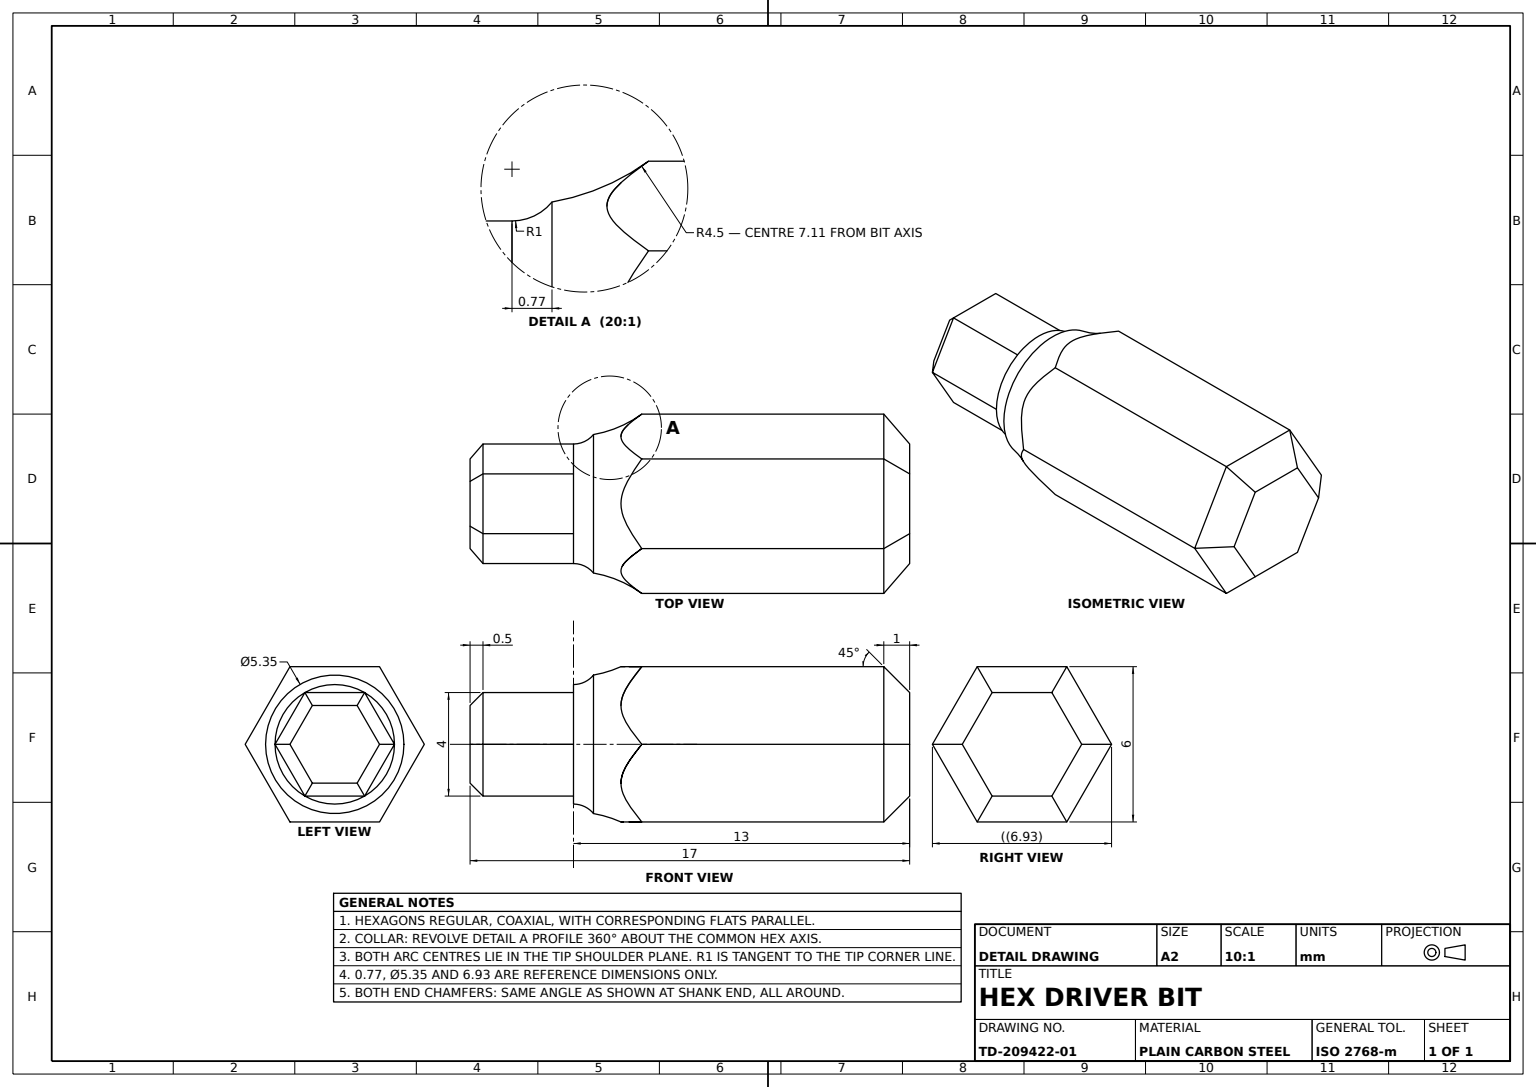
ISO-10303-21;
HEADER;
FILE_DESCRIPTION((''),'2;1');
FILE_NAME('','',(''),(''),'','','');
FILE_SCHEMA(('AUTOMOTIVE_DESIGN'));
ENDSEC;
DATA;
#1=APPLICATION_CONTEXT('');
#2=PRODUCT_CONTEXT('',#1,'mechanical');
#3=PRODUCT('','','',(#2));
#4=PRODUCT_DEFINITION_FORMATION('','',#3);
#5=PRODUCT_DEFINITION_CONTEXT('',#1,'design');
#6=PRODUCT_DEFINITION('','',#4,#5);
#7=PRODUCT_DEFINITION_SHAPE('','',#6);
#8=(LENGTH_UNIT()NAMED_UNIT(*)SI_UNIT(.MILLI.,.METRE.));
#9=(NAMED_UNIT(*)PLANE_ANGLE_UNIT()SI_UNIT($,.RADIAN.));
#10=(NAMED_UNIT(*)SI_UNIT($,.STERADIAN.)SOLID_ANGLE_UNIT());
#11=UNCERTAINTY_MEASURE_WITH_UNIT(LENGTH_MEASURE(1.E-05),#8,'distance_accuracy_value','');
#12=(GEOMETRIC_REPRESENTATION_CONTEXT(3)GLOBAL_UNCERTAINTY_ASSIGNED_CONTEXT((#11))GLOBAL_UNIT_ASSIGNED_CONTEXT((#8,#9,#10))REPRESENTATION_CONTEXT('',''));
#13=CARTESIAN_POINT('',(-2.67534,0.,12.226717));
#14=VERTEX_POINT('',#13);
#15=CARTESIAN_POINT('',(-2.309401,0.,13.));
#16=VERTEX_POINT('',#15);
#17=CARTESIAN_POINT('',(-3.309401,0.,13.));
#18=DIRECTION('',(0.,-1.,0.));
#19=DIRECTION('',(0.,0.,-1.));
#20=AXIS2_PLACEMENT_3D('',#17,#18,#19);
#21=CIRCLE('',#20,1.);
#22=EDGE_CURVE('',#14,#16,#21,.T.);
#23=ORIENTED_EDGE('',*,*,#22,.F.);
#24=CARTESIAN_POINT('',(2.67534,0.,12.226717));
#25=VERTEX_POINT('',#24);
#26=CARTESIAN_POINT('',(0.,0.,12.226717));
#27=DIRECTION('',(-1.,0.,0.));
#28=AXIS2_PLACEMENT_3D('',#26,#19,#27);
#29=CIRCLE('',#28,2.67534);
#30=EDGE_CURVE('',#25,#14,#29,.T.);
#31=ORIENTED_EDGE('',*,*,#30,.F.);
#32=CARTESIAN_POINT('',(2.309401,0.,13.));
#33=VERTEX_POINT('',#32);
#34=CARTESIAN_POINT('',(3.309401,0.,13.));
#35=DIRECTION('',(0.,1.,0.));
#36=AXIS2_PLACEMENT_3D('',#34,#35,#27);
#37=CIRCLE('',#36,1.);
#38=EDGE_CURVE('',#25,#33,#37,.T.);
#39=ORIENTED_EDGE('',*,*,#38,.T.);
#40=CARTESIAN_POINT('',(1.154701,-2.,13.));
#41=VERTEX_POINT('',#40);
#42=CARTESIAN_POINT('',(0.,0.,13.));
#43=AXIS2_PLACEMENT_3D('',#42,#19,#27);
#44=CIRCLE('',#43,2.309401);
#45=EDGE_CURVE('',#33,#41,#44,.T.);
#46=ORIENTED_EDGE('',*,*,#45,.T.);
#47=CARTESIAN_POINT('',(-1.154701,-2.,13.));
#48=VERTEX_POINT('',#47);
#49=EDGE_CURVE('',#41,#48,#44,.T.);
#50=ORIENTED_EDGE('',*,*,#49,.T.);
#51=EDGE_CURVE('',#48,#16,#44,.T.);
#52=ORIENTED_EDGE('',*,*,#51,.T.);
#53=EDGE_LOOP('',(#23,#31,#39,#46,#50,#52));
#54=FACE_OUTER_BOUND('',#53,.T.);
#55=TOROIDAL_SURFACE('',#43,3.309401,1.);
#56=ADVANCED_FACE('',(#54),#55,.F.);
#57=ORIENTED_EDGE('',*,*,#51,.F.);
#58=CARTESIAN_POINT('',(-1.732051,-1.,13.));
#59=DIRECTION('',(0.5,-0.866025404,0.));
#60=VECTOR('',#59,1000.);
#61=LINE('',#58,#60);
#62=EDGE_CURVE('',#16,#48,#61,.T.);
#63=ORIENTED_EDGE('',*,*,#62,.F.);
#64=EDGE_LOOP('',(#57,#63));
#65=FACE_OUTER_BOUND('',#64,.T.);
#66=DIRECTION('',(0.,0.,1.));
#67=DIRECTION('',(1.,0.,0.));
#68=AXIS2_PLACEMENT_3D('',#42,#66,#67);
#69=PLANE('',#68);
#70=ADVANCED_FACE('',(#65),#69,.T.);
#71=CARTESIAN_POINT('',(-0.866025,-1.5,17.));
#72=VERTEX_POINT('',#71);
#73=CARTESIAN_POINT('',(-1.154701,-2.,16.5));
#74=VERTEX_POINT('',#73);
#75=CARTESIAN_POINT('',(-0.742307,-1.285714,17.214286));
#76=DIRECTION('',(-0.377964473,-0.654653671,-0.654653671));
#77=VECTOR('',#76,1000.);
#78=LINE('',#75,#77);
#79=EDGE_CURVE('',#72,#74,#78,.T.);
#80=ORIENTED_EDGE('',*,*,#79,.F.);
#81=CARTESIAN_POINT('',(-1.732051,0.,17.));
#82=VERTEX_POINT('',#81);
#83=CARTESIAN_POINT('',(-1.299038,-0.75,17.));
#84=LINE('',#83,#60);
#85=EDGE_CURVE('',#82,#72,#84,.T.);
#86=ORIENTED_EDGE('',*,*,#85,.F.);
#87=CARTESIAN_POINT('',(-2.309401,0.,16.5));
#88=VERTEX_POINT('',#87);
#89=CARTESIAN_POINT('',(-1.484615,0.,17.214286));
#90=DIRECTION('',(-0.755928946,0.,-0.654653671));
#91=VECTOR('',#90,1000.);
#92=LINE('',#89,#91);
#93=EDGE_CURVE('',#82,#88,#92,.T.);
#94=ORIENTED_EDGE('',*,*,#93,.T.);
#95=DIRECTION('',(-0.5,0.866025404,0.));
#96=VECTOR('',#95,1000.);
#97=LINE('',#87,#96);
#98=EDGE_CURVE('',#74,#88,#97,.T.);
#99=ORIENTED_EDGE('',*,*,#98,.F.);
#100=EDGE_LOOP('',(#80,#86,#94,#99));
#101=FACE_OUTER_BOUND('',#100,.T.);
#102=DIRECTION('',(0.612372436,0.353553391,-0.707106781));
#103=AXIS2_PLACEMENT_3D('',#83,#102,#59);
#104=PLANE('',#103);
#105=ADVANCED_FACE('',(#101),#104,.F.);
#106=CARTESIAN_POINT('',(1.732051,3.,10.360098));
#107=VERTEX_POINT('',#106);
#108=CARTESIAN_POINT('',(-1.732051,3.,10.360098));
#109=VERTEX_POINT('',#108);
#110=CARTESIAN_POINT('',(1.46548,3.,10.544095));
#111=CARTESIAN_POINT('',(1.199534,3.,10.729064));
#112=CARTESIAN_POINT('',(0.772596,3.,10.962951));
#113=CARTESIAN_POINT('',(0.626195,3.,11.032542));
#114=CARTESIAN_POINT('',(0.319103,3.,11.134062));
#115=CARTESIAN_POINT('',(0.157579,3.,11.164407));
#116=CARTESIAN_POINT('',(-0.165078,3.,11.163504));
#117=CARTESIAN_POINT('',(-0.327037,3.,11.132159));
#118=CARTESIAN_POINT('',(-0.634019,3.,11.029198));
#119=CARTESIAN_POINT('',(-0.781209,3.,10.958587));
#120=CARTESIAN_POINT('',(-1.203607,3.,10.726096));
#121=CARTESIAN_POINT('',(-1.467558,3.,10.54266));
#122=B_SPLINE_CURVE_WITH_KNOTS('',3,(#106,#110,#111,#112,#113,#114,#115,#116,#117,#118,#119,#120,#121,#108),.UNSPECIFIED.,.F.,.F.,(4,2,2,2,2,2,4),(0.004347057,0.005310347,0.005791992,0.006273637,0.006755282,0.007236927,0.008200217),.UNSPECIFIED.);
#123=EDGE_CURVE('',#107,#109,#122,.T.);
#124=ORIENTED_EDGE('',*,*,#123,.F.);
#125=CARTESIAN_POINT('',(1.732051,3.,1.));
#126=VERTEX_POINT('',#125);
#127=CARTESIAN_POINT('',(1.732051,3.,13.));
#128=VECTOR('',#19,1000.);
#129=LINE('',#127,#128);
#130=EDGE_CURVE('',#107,#126,#129,.T.);
#131=ORIENTED_EDGE('',*,*,#130,.T.);
#132=CARTESIAN_POINT('',(-1.732051,3.,1.));
#133=VERTEX_POINT('',#132);
#134=VECTOR('',#27,1000.);
#135=LINE('',#125,#134);
#136=EDGE_CURVE('',#126,#133,#135,.T.);
#137=ORIENTED_EDGE('',*,*,#136,.T.);
#138=CARTESIAN_POINT('',(-1.732051,3.,13.));
#139=LINE('',#138,#128);
#140=EDGE_CURVE('',#109,#133,#139,.T.);
#141=ORIENTED_EDGE('',*,*,#140,.F.);
#142=EDGE_LOOP('',(#124,#131,#137,#141));
#143=FACE_OUTER_BOUND('',#142,.T.);
#144=AXIS2_PLACEMENT_3D('',#127,#18,#19);
#145=PLANE('',#144);
#146=ADVANCED_FACE('',(#143),#145,.F.);
#147=CARTESIAN_POINT('',(0.866025,1.5,17.));
#148=VERTEX_POINT('',#147);
#149=CARTESIAN_POINT('',(-0.866025,1.5,17.));
#150=VERTEX_POINT('',#149);
#151=CARTESIAN_POINT('',(0.,1.5,17.));
#152=LINE('',#151,#134);
#153=EDGE_CURVE('',#148,#150,#152,.T.);
#154=ORIENTED_EDGE('',*,*,#153,.F.);
#155=CARTESIAN_POINT('',(1.154701,2.,16.5));
#156=VERTEX_POINT('',#155);
#157=CARTESIAN_POINT('',(0.742307,1.285714,17.214286));
#158=DIRECTION('',(-0.377964473,-0.654653671,0.654653671));
#159=VECTOR('',#158,1000.);
#160=LINE('',#157,#159);
#161=EDGE_CURVE('',#156,#148,#160,.T.);
#162=ORIENTED_EDGE('',*,*,#161,.F.);
#163=CARTESIAN_POINT('',(-1.154701,2.,16.5));
#164=VERTEX_POINT('',#163);
#165=VECTOR('',#67,1000.);
#166=LINE('',#155,#165);
#167=EDGE_CURVE('',#164,#156,#166,.T.);
#168=ORIENTED_EDGE('',*,*,#167,.F.);
#169=CARTESIAN_POINT('',(-0.742307,1.285714,17.214286));
#170=DIRECTION('',(-0.377964473,0.654653671,-0.654653671));
#171=VECTOR('',#170,1000.);
#172=LINE('',#169,#171);
#173=EDGE_CURVE('',#150,#164,#172,.T.);
#174=ORIENTED_EDGE('',*,*,#173,.F.);
#175=EDGE_LOOP('',(#154,#162,#168,#174));
#176=FACE_OUTER_BOUND('',#175,.T.);
#177=DIRECTION('',(0.,-0.707106781,-0.707106781));
#178=AXIS2_PLACEMENT_3D('',#151,#177,#27);
#179=PLANE('',#178);
#180=ADVANCED_FACE('',(#176),#179,.F.);
#181=CARTESIAN_POINT('',(2.309401,0.,16.5));
#182=VERTEX_POINT('',#181);
#183=LINE('',#181,#60);
#184=EDGE_CURVE('',#156,#182,#183,.T.);
#185=ORIENTED_EDGE('',*,*,#184,.F.);
#186=ORIENTED_EDGE('',*,*,#161,.T.);
#187=CARTESIAN_POINT('',(1.732051,0.,17.));
#188=VERTEX_POINT('',#187);
#189=CARTESIAN_POINT('',(1.299038,0.75,17.));
#190=LINE('',#189,#96);
#191=EDGE_CURVE('',#188,#148,#190,.T.);
#192=ORIENTED_EDGE('',*,*,#191,.F.);
#193=CARTESIAN_POINT('',(1.484615,0.,17.214286));
#194=DIRECTION('',(-0.755928946,0.,0.654653671));
#195=VECTOR('',#194,1000.);
#196=LINE('',#193,#195);
#197=EDGE_CURVE('',#182,#188,#196,.T.);
#198=ORIENTED_EDGE('',*,*,#197,.F.);
#199=EDGE_LOOP('',(#185,#186,#192,#198));
#200=FACE_OUTER_BOUND('',#199,.T.);
#201=DIRECTION('',(-0.612372436,-0.353553391,-0.707106781));
#202=AXIS2_PLACEMENT_3D('',#189,#201,#95);
#203=PLANE('',#202);
#204=ADVANCED_FACE('',(#200),#203,.F.);
#205=CARTESIAN_POINT('',(-1.154701,2.,13.));
#206=VERTEX_POINT('',#205);
#207=CARTESIAN_POINT('',(-1.732051,1.,13.));
#208=DIRECTION('',(-0.5,-0.866025404,0.));
#209=VECTOR('',#208,1000.);
#210=LINE('',#207,#209);
#211=EDGE_CURVE('',#206,#16,#210,.T.);
#212=ORIENTED_EDGE('',*,*,#211,.F.);
#213=EDGE_CURVE('',#16,#206,#44,.T.);
#214=ORIENTED_EDGE('',*,*,#213,.F.);
#215=EDGE_LOOP('',(#212,#214));
#216=FACE_OUTER_BOUND('',#215,.T.);
#217=ADVANCED_FACE('',(#216),#69,.T.);
#218=CARTESIAN_POINT('',(-1.154701,2.,0.));
#219=VERTEX_POINT('',#218);
#220=CARTESIAN_POINT('',(1.154701,2.,0.));
#221=VERTEX_POINT('',#220);
#222=CARTESIAN_POINT('',(0.,2.,0.));
#223=LINE('',#222,#165);
#224=EDGE_CURVE('',#219,#221,#223,.T.);
#225=ORIENTED_EDGE('',*,*,#224,.T.);
#226=CARTESIAN_POINT('',(2.309401,0.,0.));
#227=VERTEX_POINT('',#226);
#228=CARTESIAN_POINT('',(1.732051,1.,0.));
#229=LINE('',#228,#60);
#230=EDGE_CURVE('',#221,#227,#229,.T.);
#231=ORIENTED_EDGE('',*,*,#230,.T.);
#232=CARTESIAN_POINT('',(1.154701,-2.,0.));
#233=VERTEX_POINT('',#232);
#234=CARTESIAN_POINT('',(1.732051,-1.,0.));
#235=LINE('',#234,#209);
#236=EDGE_CURVE('',#227,#233,#235,.T.);
#237=ORIENTED_EDGE('',*,*,#236,.T.);
#238=CARTESIAN_POINT('',(-1.154701,-2.,0.));
#239=VERTEX_POINT('',#238);
#240=CARTESIAN_POINT('',(0.,-2.,0.));
#241=LINE('',#240,#134);
#242=EDGE_CURVE('',#233,#239,#241,.T.);
#243=ORIENTED_EDGE('',*,*,#242,.T.);
#244=CARTESIAN_POINT('',(-2.309401,0.,0.));
#245=VERTEX_POINT('',#244);
#246=CARTESIAN_POINT('',(-1.732051,-1.,0.));
#247=LINE('',#246,#96);
#248=EDGE_CURVE('',#239,#245,#247,.T.);
#249=ORIENTED_EDGE('',*,*,#248,.T.);
#250=CARTESIAN_POINT('',(-1.732051,1.,0.));
#251=DIRECTION('',(0.5,0.866025404,0.));
#252=VECTOR('',#251,1000.);
#253=LINE('',#250,#252);
#254=EDGE_CURVE('',#245,#219,#253,.T.);
#255=ORIENTED_EDGE('',*,*,#254,.T.);
#256=EDGE_LOOP('',(#225,#231,#237,#243,#249,#255));
#257=FACE_OUTER_BOUND('',#256,.T.);
#258=CARTESIAN_POINT('',(0.,0.,0.));
#259=AXIS2_PLACEMENT_3D('',#258,#66,#67);
#260=PLANE('',#259);
#261=ADVANCED_FACE('',(#257),#260,.F.);
#262=ORIENTED_EDGE('',*,*,#173,.T.);
#263=LINE('',#163,#252);
#264=EDGE_CURVE('',#88,#164,#263,.T.);
#265=ORIENTED_EDGE('',*,*,#264,.F.);
#266=ORIENTED_EDGE('',*,*,#93,.F.);
#267=CARTESIAN_POINT('',(-1.299038,0.75,17.));
#268=LINE('',#267,#209);
#269=EDGE_CURVE('',#150,#82,#268,.T.);
#270=ORIENTED_EDGE('',*,*,#269,.F.);
#271=EDGE_LOOP('',(#262,#265,#266,#270));
#272=FACE_OUTER_BOUND('',#271,.T.);
#273=DIRECTION('',(0.612372436,-0.353553391,-0.707106781));
#274=AXIS2_PLACEMENT_3D('',#267,#273,#208);
#275=PLANE('',#274);
#276=ADVANCED_FACE('',(#272),#275,.F.);
#277=CARTESIAN_POINT('',(1.154701,-2.,16.5));
#278=VERTEX_POINT('',#277);
#279=LINE('',#277,#209);
#280=EDGE_CURVE('',#182,#278,#279,.T.);
#281=ORIENTED_EDGE('',*,*,#280,.F.);
#282=ORIENTED_EDGE('',*,*,#197,.T.);
#283=CARTESIAN_POINT('',(0.866025,-1.5,17.));
#284=VERTEX_POINT('',#283);
#285=CARTESIAN_POINT('',(1.299038,-0.75,17.));
#286=LINE('',#285,#252);
#287=EDGE_CURVE('',#284,#188,#286,.T.);
#288=ORIENTED_EDGE('',*,*,#287,.F.);
#289=CARTESIAN_POINT('',(0.742307,-1.285714,17.214286));
#290=DIRECTION('',(-0.377964473,0.654653671,0.654653671));
#291=VECTOR('',#290,1000.);
#292=LINE('',#289,#291);
#293=EDGE_CURVE('',#278,#284,#292,.T.);
#294=ORIENTED_EDGE('',*,*,#293,.F.);
#295=EDGE_LOOP('',(#281,#282,#288,#294));
#296=FACE_OUTER_BOUND('',#295,.T.);
#297=DIRECTION('',(-0.612372436,0.353553391,-0.707106781));
#298=AXIS2_PLACEMENT_3D('',#285,#297,#251);
#299=PLANE('',#298);
#300=ADVANCED_FACE('',(#296),#299,.F.);
#301=CARTESIAN_POINT('',(-1.732051,-3.,10.360098));
#302=VERTEX_POINT('',#301);
#303=CARTESIAN_POINT('',(1.732051,-3.,10.360098));
#304=VERTEX_POINT('',#303);
#305=CARTESIAN_POINT('',(-1.46548,-3.,10.544095));
#306=CARTESIAN_POINT('',(-1.199534,-3.,10.729064));
#307=CARTESIAN_POINT('',(-0.772596,-3.,10.962951));
#308=CARTESIAN_POINT('',(-0.626195,-3.,11.032542));
#309=CARTESIAN_POINT('',(-0.319103,-3.,11.134062));
#310=CARTESIAN_POINT('',(-0.157579,-3.,11.164407));
#311=CARTESIAN_POINT('',(0.165078,-3.,11.163504));
#312=CARTESIAN_POINT('',(0.327037,-3.,11.132159));
#313=CARTESIAN_POINT('',(0.634019,-3.,11.029198));
#314=CARTESIAN_POINT('',(0.781209,-3.,10.958587));
#315=CARTESIAN_POINT('',(1.203607,-3.,10.726096));
#316=CARTESIAN_POINT('',(1.467558,-3.,10.54266));
#317=B_SPLINE_CURVE_WITH_KNOTS('',3,(#301,#305,#306,#307,#308,#309,#310,#311,#312,#313,#314,#315,#316,#303),.UNSPECIFIED.,.F.,.F.,(4,2,2,2,2,2,4),(0.004347057,0.005310347,0.005791992,0.006273637,0.006755282,0.007236927,0.008200217),.UNSPECIFIED.);
#318=EDGE_CURVE('',#302,#304,#317,.T.);
#319=ORIENTED_EDGE('',*,*,#318,.F.);
#320=CARTESIAN_POINT('',(-1.732051,-3.,1.));
#321=VERTEX_POINT('',#320);
#322=CARTESIAN_POINT('',(-1.732051,-3.,13.));
#323=LINE('',#322,#128);
#324=EDGE_CURVE('',#302,#321,#323,.T.);
#325=ORIENTED_EDGE('',*,*,#324,.T.);
#326=CARTESIAN_POINT('',(1.732051,-3.,1.));
#327=VERTEX_POINT('',#326);
#328=LINE('',#320,#165);
#329=EDGE_CURVE('',#321,#327,#328,.T.);
#330=ORIENTED_EDGE('',*,*,#329,.T.);
#331=CARTESIAN_POINT('',(1.732051,-3.,13.));
#332=LINE('',#331,#128);
#333=EDGE_CURVE('',#304,#327,#332,.T.);
#334=ORIENTED_EDGE('',*,*,#333,.F.);
#335=EDGE_LOOP('',(#319,#325,#330,#334));
#336=FACE_OUTER_BOUND('',#335,.T.);
#337=AXIS2_PLACEMENT_3D('',#322,#35,#66);
#338=PLANE('',#337);
#339=ADVANCED_FACE('',(#336),#338,.F.);
#340=CARTESIAN_POINT('',(1.154701,2.,13.));
#341=VERTEX_POINT('',#340);
#342=EDGE_CURVE('',#341,#33,#44,.T.);
#343=ORIENTED_EDGE('',*,*,#342,.F.);
#344=CARTESIAN_POINT('',(1.732051,1.,13.));
#345=LINE('',#344,#96);
#346=EDGE_CURVE('',#33,#341,#345,.T.);
#347=ORIENTED_EDGE('',*,*,#346,.F.);
#348=EDGE_LOOP('',(#343,#347));
#349=FACE_OUTER_BOUND('',#348,.T.);
#350=ADVANCED_FACE('',(#349),#69,.T.);
#351=CARTESIAN_POINT('',(-3.464102,0.,10.360098));
#352=VERTEX_POINT('',#351);
#353=CARTESIAN_POINT('',(-1.865194,2.76939,10.543898));
#354=CARTESIAN_POINT('',(-1.99824,2.538946,10.728897));
#355=CARTESIAN_POINT('',(-2.211152,2.170172,10.96231));
#356=CARTESIAN_POINT('',(-2.283891,2.044184,11.031576));
#357=CARTESIAN_POINT('',(-2.436992,1.779005,11.133292));
#358=CARTESIAN_POINT('',(-2.517802,1.639038,11.164022));
#359=CARTESIAN_POINT('',(-2.678865,1.360069,11.163899));
#360=CARTESIAN_POINT('',(-2.759942,1.219639,11.132945));
#361=CARTESIAN_POINT('',(-2.913333,0.953959,11.030688));
#362=CARTESIAN_POINT('',(-2.987069,0.826245,10.960215));
#363=CARTESIAN_POINT('',(-3.198866,0.459402,10.7275));
#364=CARTESIAN_POINT('',(-3.331351,0.229931,10.543357));
#365=B_SPLINE_CURVE_WITH_KNOTS('',3,(#108,#353,#354,#355,#356,#357,#358,#359,#360,#361,#362,#363,#364,#351),.UNSPECIFIED.,.F.,.F.,(4,2,2,2,2,2,4),(0.00000028,0.000970506,0.001455618,0.001940731,0.002425844,0.002910956,0.003881181),.UNSPECIFIED.);
#366=EDGE_CURVE('',#109,#352,#365,.T.);
#367=ORIENTED_EDGE('',*,*,#366,.T.);
#368=CARTESIAN_POINT('',(-7.108401,0.,13.));
#369=AXIS2_PLACEMENT_3D('',#368,#18,#19);
#370=CIRCLE('',#369,4.5);
#371=EDGE_CURVE('',#352,#14,#370,.T.);
#372=ORIENTED_EDGE('',*,*,#371,.T.);
#373=EDGE_CURVE('',#14,#25,#29,.T.);
#374=ORIENTED_EDGE('',*,*,#373,.T.);
#375=CARTESIAN_POINT('',(3.464102,0.,10.360098));
#376=VERTEX_POINT('',#375);
#377=CARTESIAN_POINT('',(7.108401,0.,13.));
#378=AXIS2_PLACEMENT_3D('',#377,#35,#27);
#379=CIRCLE('',#378,4.5);
#380=EDGE_CURVE('',#376,#25,#379,.T.);
#381=ORIENTED_EDGE('',*,*,#380,.F.);
#382=CARTESIAN_POINT('',(3.330959,0.23061,10.543898));
#383=CARTESIAN_POINT('',(3.197912,0.461054,10.728897));
#384=CARTESIAN_POINT('',(2.985,0.829828,10.96231));
#385=CARTESIAN_POINT('',(2.912261,0.955816,11.031576));
#386=CARTESIAN_POINT('',(2.75916,1.220995,11.133292));
#387=CARTESIAN_POINT('',(2.67835,1.360962,11.164022));
#388=CARTESIAN_POINT('',(2.517287,1.639931,11.163899));
#389=CARTESIAN_POINT('',(2.43621,1.780361,11.132945));
#390=CARTESIAN_POINT('',(2.282819,2.046041,11.030688));
#391=CARTESIAN_POINT('',(2.209083,2.173755,10.960215));
#392=CARTESIAN_POINT('',(1.997287,2.540598,10.7275));
#393=CARTESIAN_POINT('',(1.864802,2.770069,10.543357));
#394=B_SPLINE_CURVE_WITH_KNOTS('',3,(#375,#382,#383,#384,#385,#386,#387,#388,#389,#390,#391,#392,#393,#106),.UNSPECIFIED.,.F.,.F.,(4,2,2,2,2,2,4),(0.00000028,0.000970506,0.001455618,0.001940731,0.002425844,0.002910956,0.003881181),.UNSPECIFIED.);
#395=EDGE_CURVE('',#376,#107,#394,.T.);
#396=ORIENTED_EDGE('',*,*,#395,.T.);
#397=ORIENTED_EDGE('',*,*,#123,.T.);
#398=EDGE_LOOP('',(#367,#372,#374,#381,#396,#397));
#399=FACE_OUTER_BOUND('',#398,.T.);
#400=TOROIDAL_SURFACE('',#43,7.108401,4.5);
#401=ADVANCED_FACE('',(#399),#400,.F.);
#402=CARTESIAN_POINT('',(-1.154701,-2.,9.));
#403=VECTOR('',#66,1000.);
#404=LINE('',#402,#403);
#405=EDGE_CURVE('',#48,#74,#404,.T.);
#406=ORIENTED_EDGE('',*,*,#405,.T.);
#407=ORIENTED_EDGE('',*,*,#98,.T.);
#408=CARTESIAN_POINT('',(-2.309401,0.,9.));
#409=LINE('',#408,#403);
#410=EDGE_CURVE('',#16,#88,#409,.T.);
#411=ORIENTED_EDGE('',*,*,#410,.F.);
#412=ORIENTED_EDGE('',*,*,#62,.T.);
#413=EDGE_LOOP('',(#406,#407,#411,#412));
#414=FACE_OUTER_BOUND('',#413,.T.);
#415=DIRECTION('',(-0.866025404,-0.5,0.));
#416=AXIS2_PLACEMENT_3D('',#408,#415,#59);
#417=PLANE('',#416);
#418=ADVANCED_FACE('',(#414),#417,.T.);
#419=ORIENTED_EDGE('',*,*,#136,.F.);
#420=DIRECTION('',(0.377964473,0.654653671,0.654653671));
#421=VECTOR('',#420,1000.);
#422=LINE('',#125,#421);
#423=EDGE_CURVE('',#221,#126,#422,.T.);
#424=ORIENTED_EDGE('',*,*,#423,.F.);
#425=ORIENTED_EDGE('',*,*,#224,.F.);
#426=LINE('',#132,#291);
#427=EDGE_CURVE('',#219,#133,#426,.T.);
#428=ORIENTED_EDGE('',*,*,#427,.T.);
#429=EDGE_LOOP('',(#419,#424,#425,#428));
#430=FACE_OUTER_BOUND('',#429,.T.);
#431=DIRECTION('',(0.,-0.707106781,0.707106781));
#432=AXIS2_PLACEMENT_3D('',#125,#431,#27);
#433=PLANE('',#432);
#434=ADVANCED_FACE('',(#430),#433,.F.);
#435=CARTESIAN_POINT('',(3.464102,0.,1.));
#436=VERTEX_POINT('',#435);
#437=LINE('',#326,#252);
#438=EDGE_CURVE('',#327,#436,#437,.T.);
#439=ORIENTED_EDGE('',*,*,#438,.T.);
#440=CARTESIAN_POINT('',(3.464102,0.,13.));
#441=LINE('',#440,#128);
#442=EDGE_CURVE('',#376,#436,#441,.T.);
#443=ORIENTED_EDGE('',*,*,#442,.F.);
#444=CARTESIAN_POINT('',(1.865194,-2.76939,10.543898));
#445=CARTESIAN_POINT('',(1.99824,-2.538946,10.728897));
#446=CARTESIAN_POINT('',(2.211152,-2.170172,10.96231));
#447=CARTESIAN_POINT('',(2.283891,-2.044184,11.031576));
#448=CARTESIAN_POINT('',(2.436992,-1.779005,11.133292));
#449=CARTESIAN_POINT('',(2.517802,-1.639038,11.164022));
#450=CARTESIAN_POINT('',(2.678865,-1.360069,11.163899));
#451=CARTESIAN_POINT('',(2.759942,-1.219639,11.132945));
#452=CARTESIAN_POINT('',(2.913333,-0.953959,11.030688));
#453=CARTESIAN_POINT('',(2.987069,-0.826245,10.960215));
#454=CARTESIAN_POINT('',(3.198866,-0.459402,10.7275));
#455=CARTESIAN_POINT('',(3.331351,-0.229931,10.543357));
#456=B_SPLINE_CURVE_WITH_KNOTS('',3,(#303,#444,#445,#446,#447,#448,#449,#450,#451,#452,#453,#454,#455,#375),.UNSPECIFIED.,.F.,.F.,(4,2,2,2,2,2,4),(0.00000028,0.000970506,0.001455618,0.001940731,0.002425844,0.002910956,0.003881181),.UNSPECIFIED.);
#457=EDGE_CURVE('',#304,#376,#456,.T.);
#458=ORIENTED_EDGE('',*,*,#457,.F.);
#459=ORIENTED_EDGE('',*,*,#333,.T.);
#460=EDGE_LOOP('',(#439,#443,#458,#459));
#461=FACE_OUTER_BOUND('',#460,.T.);
#462=DIRECTION('',(-0.866025404,0.5,0.));
#463=AXIS2_PLACEMENT_3D('',#331,#462,#208);
#464=PLANE('',#463);
#465=ADVANCED_FACE('',(#461),#464,.F.);
#466=ORIENTED_EDGE('',*,*,#329,.F.);
#467=DIRECTION('',(0.377964473,0.654653671,-0.654653671));
#468=VECTOR('',#467,1000.);
#469=LINE('',#320,#468);
#470=EDGE_CURVE('',#321,#239,#469,.T.);
#471=ORIENTED_EDGE('',*,*,#470,.T.);
#472=ORIENTED_EDGE('',*,*,#242,.F.);
#473=LINE('',#326,#171);
#474=EDGE_CURVE('',#327,#233,#473,.T.);
#475=ORIENTED_EDGE('',*,*,#474,.F.);
#476=EDGE_LOOP('',(#466,#471,#472,#475));
#477=FACE_OUTER_BOUND('',#476,.T.);
#478=DIRECTION('',(0.,0.707106781,0.707106781));
#479=AXIS2_PLACEMENT_3D('',#320,#478,#67);
#480=PLANE('',#479);
#481=ADVANCED_FACE('',(#477),#480,.F.);
#482=ORIENTED_EDGE('',*,*,#427,.F.);
#483=ORIENTED_EDGE('',*,*,#254,.F.);
#484=CARTESIAN_POINT('',(-3.464102,0.,1.));
#485=VERTEX_POINT('',#484);
#486=LINE('',#484,#195);
#487=EDGE_CURVE('',#245,#485,#486,.T.);
#488=ORIENTED_EDGE('',*,*,#487,.T.);
#489=LINE('',#132,#209);
#490=EDGE_CURVE('',#133,#485,#489,.T.);
#491=ORIENTED_EDGE('',*,*,#490,.F.);
#492=EDGE_LOOP('',(#482,#483,#488,#491));
#493=FACE_OUTER_BOUND('',#492,.T.);
#494=DIRECTION('',(0.612372436,-0.353553391,0.707106781));
#495=AXIS2_PLACEMENT_3D('',#132,#494,#208);
#496=PLANE('',#495);
#497=ADVANCED_FACE('',(#493),#496,.F.);
#498=ORIENTED_EDGE('',*,*,#474,.T.);
#499=ORIENTED_EDGE('',*,*,#236,.F.);
#500=CARTESIAN_POINT('',(2.474358,0.,0.142857));
#501=LINE('',#500,#91);
#502=EDGE_CURVE('',#436,#227,#501,.T.);
#503=ORIENTED_EDGE('',*,*,#502,.F.);
#504=ORIENTED_EDGE('',*,*,#438,.F.);
#505=EDGE_LOOP('',(#498,#499,#503,#504));
#506=FACE_OUTER_BOUND('',#505,.T.);
#507=DIRECTION('',(-0.612372436,0.353553391,0.707106781));
#508=AXIS2_PLACEMENT_3D('',#326,#507,#251);
#509=PLANE('',#508);
#510=ADVANCED_FACE('',(#506),#509,.F.);
#511=ORIENTED_EDGE('',*,*,#167,.T.);
#512=CARTESIAN_POINT('',(1.154701,2.,9.));
#513=LINE('',#512,#403);
#514=EDGE_CURVE('',#341,#156,#513,.T.);
#515=ORIENTED_EDGE('',*,*,#514,.F.);
#516=CARTESIAN_POINT('',(0.,2.,13.));
#517=LINE('',#516,#134);
#518=EDGE_CURVE('',#341,#206,#517,.T.);
#519=ORIENTED_EDGE('',*,*,#518,.T.);
#520=CARTESIAN_POINT('',(-1.154701,2.,9.));
#521=LINE('',#520,#403);
#522=EDGE_CURVE('',#206,#164,#521,.T.);
#523=ORIENTED_EDGE('',*,*,#522,.T.);
#524=EDGE_LOOP('',(#511,#515,#519,#523));
#525=FACE_OUTER_BOUND('',#524,.T.);
#526=AXIS2_PLACEMENT_3D('',#512,#35,#66);
#527=PLANE('',#526);
#528=ADVANCED_FACE('',(#525),#527,.T.);
#529=ORIENTED_EDGE('',*,*,#85,.T.);
#530=CARTESIAN_POINT('',(0.,-1.5,17.));
#531=LINE('',#530,#165);
#532=EDGE_CURVE('',#72,#284,#531,.T.);
#533=ORIENTED_EDGE('',*,*,#532,.T.);
#534=ORIENTED_EDGE('',*,*,#287,.T.);
#535=ORIENTED_EDGE('',*,*,#191,.T.);
#536=ORIENTED_EDGE('',*,*,#153,.T.);
#537=ORIENTED_EDGE('',*,*,#269,.T.);
#538=EDGE_LOOP('',(#529,#533,#534,#535,#536,#537));
#539=FACE_OUTER_BOUND('',#538,.T.);
#540=CARTESIAN_POINT('',(0.,0.,17.));
#541=AXIS2_PLACEMENT_3D('',#540,#66,#67);
#542=PLANE('',#541);
#543=ADVANCED_FACE('',(#539),#542,.T.);
#544=CARTESIAN_POINT('',(-3.464102,0.,13.));
#545=LINE('',#544,#128);
#546=EDGE_CURVE('',#352,#485,#545,.T.);
#547=ORIENTED_EDGE('',*,*,#546,.F.);
#548=ORIENTED_EDGE('',*,*,#366,.F.);
#549=ORIENTED_EDGE('',*,*,#140,.T.);
#550=ORIENTED_EDGE('',*,*,#490,.T.);
#551=EDGE_LOOP('',(#547,#548,#549,#550));
#552=FACE_OUTER_BOUND('',#551,.T.);
#553=DIRECTION('',(0.866025404,-0.5,0.));
#554=AXIS2_PLACEMENT_3D('',#138,#553,#251);
#555=PLANE('',#554);
#556=ADVANCED_FACE('',(#552),#555,.F.);
#557=ORIENTED_EDGE('',*,*,#342,.T.);
#558=ORIENTED_EDGE('',*,*,#38,.F.);
#559=ORIENTED_EDGE('',*,*,#373,.F.);
#560=ORIENTED_EDGE('',*,*,#22,.T.);
#561=ORIENTED_EDGE('',*,*,#213,.T.);
#562=EDGE_CURVE('',#206,#341,#44,.T.);
#563=ORIENTED_EDGE('',*,*,#562,.T.);
#564=EDGE_LOOP('',(#557,#558,#559,#560,#561,#563));
#565=FACE_OUTER_BOUND('',#564,.T.);
#566=ADVANCED_FACE('',(#565),#55,.F.);
#567=ORIENTED_EDGE('',*,*,#45,.F.);
#568=CARTESIAN_POINT('',(1.732051,-1.,13.));
#569=LINE('',#568,#252);
#570=EDGE_CURVE('',#41,#33,#569,.T.);
#571=ORIENTED_EDGE('',*,*,#570,.F.);
#572=EDGE_LOOP('',(#567,#571));
#573=FACE_OUTER_BOUND('',#572,.T.);
#574=ADVANCED_FACE('',(#573),#69,.T.);
#575=ORIENTED_EDGE('',*,*,#79,.T.);
#576=LINE('',#73,#134);
#577=EDGE_CURVE('',#278,#74,#576,.T.);
#578=ORIENTED_EDGE('',*,*,#577,.F.);
#579=ORIENTED_EDGE('',*,*,#293,.T.);
#580=ORIENTED_EDGE('',*,*,#532,.F.);
#581=EDGE_LOOP('',(#575,#578,#579,#580));
#582=FACE_OUTER_BOUND('',#581,.T.);
#583=DIRECTION('',(0.,0.707106781,-0.707106781));
#584=AXIS2_PLACEMENT_3D('',#530,#583,#67);
#585=PLANE('',#584);
#586=ADVANCED_FACE('',(#582),#585,.F.);
#587=CARTESIAN_POINT('',(0.,-2.,13.));
#588=LINE('',#587,#165);
#589=EDGE_CURVE('',#48,#41,#588,.T.);
#590=ORIENTED_EDGE('',*,*,#589,.F.);
#591=ORIENTED_EDGE('',*,*,#49,.F.);
#592=EDGE_LOOP('',(#590,#591));
#593=FACE_OUTER_BOUND('',#592,.T.);
#594=ADVANCED_FACE('',(#593),#69,.T.);
#595=ORIENTED_EDGE('',*,*,#487,.F.);
#596=ORIENTED_EDGE('',*,*,#248,.F.);
#597=ORIENTED_EDGE('',*,*,#470,.F.);
#598=LINE('',#484,#60);
#599=EDGE_CURVE('',#485,#321,#598,.T.);
#600=ORIENTED_EDGE('',*,*,#599,.F.);
#601=EDGE_LOOP('',(#595,#596,#597,#600));
#602=FACE_OUTER_BOUND('',#601,.T.);
#603=DIRECTION('',(0.612372436,0.353553391,0.707106781));
#604=AXIS2_PLACEMENT_3D('',#484,#603,#59);
#605=PLANE('',#604);
#606=ADVANCED_FACE('',(#602),#605,.F.);
#607=ORIENTED_EDGE('',*,*,#546,.T.);
#608=ORIENTED_EDGE('',*,*,#599,.T.);
#609=ORIENTED_EDGE('',*,*,#324,.F.);
#610=CARTESIAN_POINT('',(-3.330959,-0.23061,10.543898));
#611=CARTESIAN_POINT('',(-3.197912,-0.461054,10.728897));
#612=CARTESIAN_POINT('',(-2.985,-0.829828,10.96231));
#613=CARTESIAN_POINT('',(-2.912261,-0.955816,11.031576));
#614=CARTESIAN_POINT('',(-2.75916,-1.220995,11.133292));
#615=CARTESIAN_POINT('',(-2.67835,-1.360962,11.164022));
#616=CARTESIAN_POINT('',(-2.517287,-1.639931,11.163899));
#617=CARTESIAN_POINT('',(-2.43621,-1.780361,11.132945));
#618=CARTESIAN_POINT('',(-2.282819,-2.046041,11.030688));
#619=CARTESIAN_POINT('',(-2.209083,-2.173755,10.960215));
#620=CARTESIAN_POINT('',(-1.997287,-2.540598,10.7275));
#621=CARTESIAN_POINT('',(-1.864802,-2.770069,10.543357));
#622=B_SPLINE_CURVE_WITH_KNOTS('',3,(#351,#610,#611,#612,#613,#614,#615,#616,#617,#618,#619,#620,#621,#301),.UNSPECIFIED.,.F.,.F.,(4,2,2,2,2,2,4),(0.00000028,0.000970506,0.001455618,0.001940731,0.002425844,0.002910956,0.003881181),.UNSPECIFIED.);
#623=EDGE_CURVE('',#352,#302,#622,.T.);
#624=ORIENTED_EDGE('',*,*,#623,.F.);
#625=EDGE_LOOP('',(#607,#608,#609,#624));
#626=FACE_OUTER_BOUND('',#625,.T.);
#627=DIRECTION('',(0.866025404,0.5,0.));
#628=AXIS2_PLACEMENT_3D('',#544,#627,#95);
#629=PLANE('',#628);
#630=ADVANCED_FACE('',(#626),#629,.F.);
#631=ORIENTED_EDGE('',*,*,#410,.T.);
#632=ORIENTED_EDGE('',*,*,#264,.T.);
#633=ORIENTED_EDGE('',*,*,#522,.F.);
#634=ORIENTED_EDGE('',*,*,#211,.T.);
#635=EDGE_LOOP('',(#631,#632,#633,#634));
#636=FACE_OUTER_BOUND('',#635,.T.);
#637=AXIS2_PLACEMENT_3D('',#520,#462,#208);
#638=PLANE('',#637);
#639=ADVANCED_FACE('',(#636),#638,.T.);
#640=ORIENTED_EDGE('',*,*,#589,.T.);
#641=CARTESIAN_POINT('',(1.154701,-2.,9.));
#642=LINE('',#641,#403);
#643=EDGE_CURVE('',#41,#278,#642,.T.);
#644=ORIENTED_EDGE('',*,*,#643,.T.);
#645=ORIENTED_EDGE('',*,*,#577,.T.);
#646=ORIENTED_EDGE('',*,*,#405,.F.);
#647=EDGE_LOOP('',(#640,#644,#645,#646));
#648=FACE_OUTER_BOUND('',#647,.T.);
#649=AXIS2_PLACEMENT_3D('',#402,#18,#19);
#650=PLANE('',#649);
#651=ADVANCED_FACE('',(#648),#650,.T.);
#652=ORIENTED_EDGE('',*,*,#442,.T.);
#653=LINE('',#435,#96);
#654=EDGE_CURVE('',#436,#126,#653,.T.);
#655=ORIENTED_EDGE('',*,*,#654,.T.);
#656=ORIENTED_EDGE('',*,*,#130,.F.);
#657=ORIENTED_EDGE('',*,*,#395,.F.);
#658=EDGE_LOOP('',(#652,#655,#656,#657));
#659=FACE_OUTER_BOUND('',#658,.T.);
#660=AXIS2_PLACEMENT_3D('',#440,#415,#59);
#661=PLANE('',#660);
#662=ADVANCED_FACE('',(#659),#661,.F.);
#663=ORIENTED_EDGE('',*,*,#623,.T.);
#664=ORIENTED_EDGE('',*,*,#318,.T.);
#665=ORIENTED_EDGE('',*,*,#457,.T.);
#666=ORIENTED_EDGE('',*,*,#380,.T.);
#667=ORIENTED_EDGE('',*,*,#30,.T.);
#668=ORIENTED_EDGE('',*,*,#371,.F.);
#669=EDGE_LOOP('',(#663,#664,#665,#666,#667,#668));
#670=FACE_OUTER_BOUND('',#669,.T.);
#671=ADVANCED_FACE('',(#670),#400,.F.);
#672=ORIENTED_EDGE('',*,*,#643,.F.);
#673=ORIENTED_EDGE('',*,*,#570,.T.);
#674=CARTESIAN_POINT('',(2.309401,0.,9.));
#675=LINE('',#674,#403);
#676=EDGE_CURVE('',#33,#182,#675,.T.);
#677=ORIENTED_EDGE('',*,*,#676,.T.);
#678=ORIENTED_EDGE('',*,*,#280,.T.);
#679=EDGE_LOOP('',(#672,#673,#677,#678));
#680=FACE_OUTER_BOUND('',#679,.T.);
#681=AXIS2_PLACEMENT_3D('',#641,#553,#251);
#682=PLANE('',#681);
#683=ADVANCED_FACE('',(#680),#682,.T.);
#684=ORIENTED_EDGE('',*,*,#346,.T.);
#685=ORIENTED_EDGE('',*,*,#514,.T.);
#686=ORIENTED_EDGE('',*,*,#184,.T.);
#687=ORIENTED_EDGE('',*,*,#676,.F.);
#688=EDGE_LOOP('',(#684,#685,#686,#687));
#689=FACE_OUTER_BOUND('',#688,.T.);
#690=AXIS2_PLACEMENT_3D('',#674,#627,#95);
#691=PLANE('',#690);
#692=ADVANCED_FACE('',(#689),#691,.T.);
#693=ORIENTED_EDGE('',*,*,#562,.F.);
#694=ORIENTED_EDGE('',*,*,#518,.F.);
#695=EDGE_LOOP('',(#693,#694));
#696=FACE_OUTER_BOUND('',#695,.T.);
#697=ADVANCED_FACE('',(#696),#69,.T.);
#698=ORIENTED_EDGE('',*,*,#654,.F.);
#699=ORIENTED_EDGE('',*,*,#502,.T.);
#700=ORIENTED_EDGE('',*,*,#230,.F.);
#701=ORIENTED_EDGE('',*,*,#423,.T.);
#702=EDGE_LOOP('',(#698,#699,#700,#701));
#703=FACE_OUTER_BOUND('',#702,.T.);
#704=DIRECTION('',(-0.612372436,-0.353553391,0.707106781));
#705=AXIS2_PLACEMENT_3D('',#435,#704,#95);
#706=PLANE('',#705);
#707=ADVANCED_FACE('',(#703),#706,.F.);
#708=CLOSED_SHELL('',(#56,#70,#105,#146,#180,#204,#217,#261,#276,#300,#339,#350,#401,#418,#434,#465,#481,#497,#510,#528,#543,#556,#566,#574,#586,#594,#606,#630,#639,#651,#662,#671,#683,#692,#697,#707));
#709=MANIFOLD_SOLID_BREP('',#708);
#710=ADVANCED_BREP_SHAPE_REPRESENTATION('',(#709),#12);
#711=SHAPE_DEFINITION_REPRESENTATION(#7,#710);
ENDSEC;
END-ISO-10303-21;
